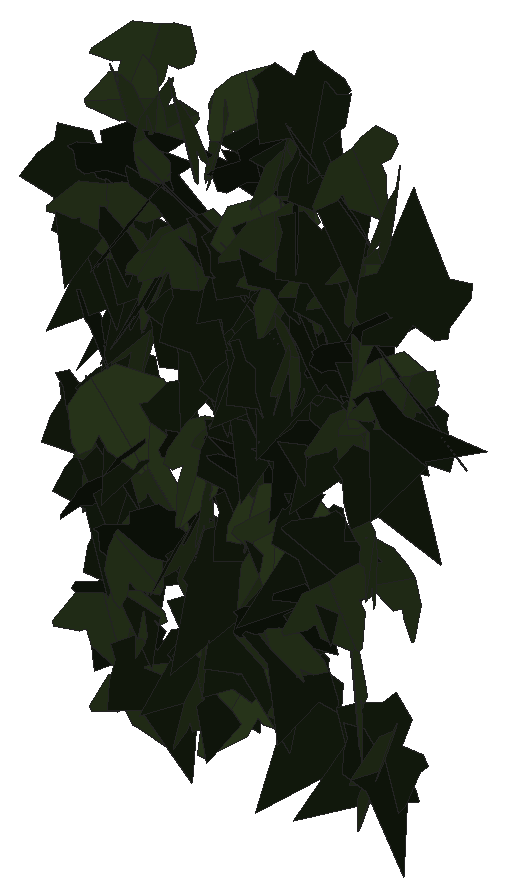
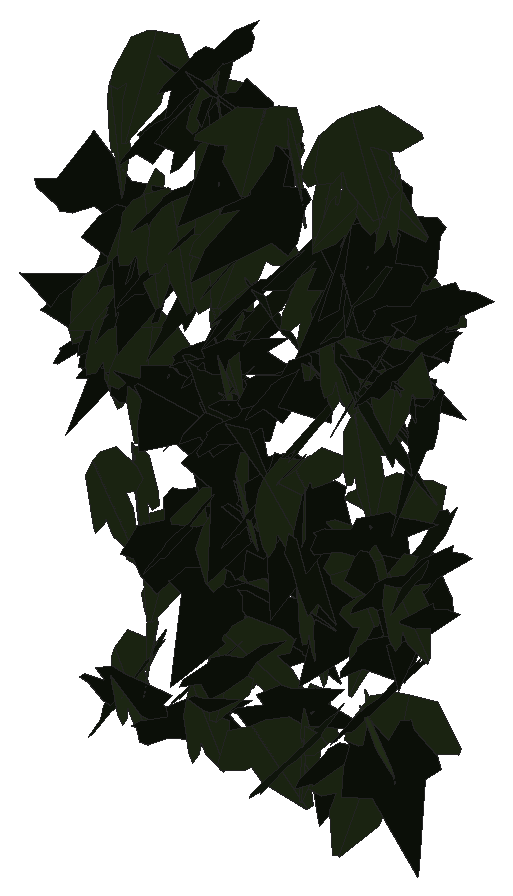
# SketchUp Ruby script. Lengths in inches.
U = 1.inch
M = Sketchup.active_model
def pt(a) = Geom::Point3d.new(a.map { |v| v * U })
def face(e, loops, mat)
  f = e.add_face(loops[0].map { |a| pt(a) })
  loops[1..].each { |l| e.add_face(l.map { |a| pt(a) }).erase! }
  f.material = f.back_material = mat if mat
  f
end
# faces: each face lists its corners as indices into pts; further lists are holes
def faces(e, pts, list, mat = nil) = list.each { |f| face(e, (f[0].is_a?(Array) ? f : [f]).map { |l| l.map { |i| pts[i] } }, mat) }
# xy, xz, yz: faces in a plane at the given z, y or x. An outline is a flat list of corners, or four numbers for a rectangle; further outlines are holes
def ring(l) = l.size == 4 ? [[l[0], l[1]], [l[2], l[1]], [l[2], l[3]], [l[0], l[3]]] : l.each_slice(2).to_a
def flat(e, list, mat, &to3) = list.each { |f| face(e, (f[0].is_a?(Array) ? f : [f]).map { |l| ring(l).map { |u, v| to3.(u, v) } }, mat) }
def xy(e, z, list, mat = nil) = flat(e, list, mat) { |x, y| [x, y, z] }
def xz(e, y, list, mat = nil) = flat(e, list, mat) { |x, z| [x, y, z] }
def yz(e, x, list, mat = nil) = flat(e, list, mat) { |y, z| [x, y, z] }
def lines(e, pts, list) = list.each { |a, b| e.add_line(pt(pts[a]), pt(pts[b])) }
# prism: a flat outline (further loops are holes) pulled along v
def prism(e, loops, v, mat = nil)
  f = face(e, loops, mat); d = Geom::Vector3d.new(v.map { |x| x * U })
  f.pushpull(f.normal.samedirection?(d) ? d.length : -d.length)
end
def box(e, o, s, mat = nil) = prism(e, [[o, [o[0] + s[0], o[1], o[2]], [o[0] + s[0], o[1] + s[1], o[2]], [o[0], o[1] + s[1], o[2]]]], [0, 0, s[2]], mat)
def at(x, y, z, deg = 0) = Geom::Transformation.translation(pt([x, y, z])) * Geom::Transformation.rotation(ORIGIN, Z_AXIS, deg.degrees)
def axes(o, x, y, z) = Geom::Transformation.new([*x, 0, *y, 0, *z, 0, *pt(o).to_a, 1])
def part(name) = M.definitions.add(name)
# library, detail: a bought-in or finely detailed component or shape, given as its bounding box
def library(name, o, s) = part(name).tap { |d| box(d.entities, o, s) }
def detail(e, o, s) = box(e.add_group.entities, o, s)
def put(e, d, t, mat = nil) = e.add_instance(d, t).tap { |i| i.material = mat if mat }
def group(e, t, mat = nil) = e.add_group.tap { |g| g.transformation = t; g.material = mat if mat }.entities
root = M.entities
M.materials.add("efeu1").color = [18, 25, 13]
M.materials.add("efeu2").color = [43, 57, 29]
c1 = part("ivyleaf_9")
p = [[1.54,2.16,1.25],[1.36,2.04,1.19],[-0.21,0.99,0.68],[-0.71,1.11,0.82],[-0.85,0.86,0.67],[-0.8,0.17,0.21],
  [-0.9,-0.01,0.1],[-0.67,-0.16,-0.02],[-0.08,-0.08,-0.05],[-0.03,-0.6,-0.4],[0.65,-0.88,-0.66],[0.83,-0.6,-0.49],
  [1.29,-0.42,-0.43],[1.8125,-0.07,-0.26],[1.21,0.44,0.15]]
faces(c1.entities,p,[[0,1,2,3,4,5,6,7,8,9,10,11,12,13,14]],"efeu1")
c2 = part("ivyleaf_10")
p = [[0,0.5,-0.03],[-0.0625,2.02,-0.43],[-0.19,2.01,-0.46],[-0.54,1.05,-0.29],[-0.52,0.625,-0.18],[-0.83,0.76,-0.28],
  [-1.16,0.64,-0.33],[-1.15,0.33,-0.24],[-0.77,-0.39,0.02],[-0.3,-0.51,0.16],[0.04,-0.48,0.23],[-0.02,2.01,-0.4375],
  [-0.06,2.01,-0.43],[0.04,-0.49,0.23],[0.67,-0.49,0.14],[1.38,0.36,-0.2],[1.375,0.51,-0.24],[0.81,0.65,-0.19],
  [0.62,0.59,-0.15],[0.6,1.09,-0.28],[0.5,1.23,-0.31]]
faces(c2.entities,p,[[0,1,2,3,4,5,6,7,8,9,10],[11,12,0,13,14,15,16,17,18,19,20]],"efeu2")
put(root,c1,axes([37.34,222.2,235.97],[0.37722,0.32248,0.06095],[0.04735,0.03841,-0.49627],[-0.32475,0.38018,-0.00156]))
put(root,c1,axes([39.04,222.6,238.55],[0.0869,-0.47634,-0.12469],[-0.01541,0.12393,-0.48415],[0.49215,0.08798,0.00686]))
put(root,c1,axes([37.5,222.54,239.24],[-0.33451,0.31048,-0.20422],[0.14578,-0.14311,-0.45636],[-0.34183,-0.36486,0.00522]))
put(root,c2,axes([38.09,222.62,237.15],[0.16547,0.41655,-0.22161],[-0.1056,-0.19618,-0.44762],[-0.45986,0.19494,0.02305]))
put(root,c1,axes([40.66,222.42,237.91],[0.16946,-0.36104,-0.30155],[-0.07838,0.29437,-0.39649],[0.46383,0.18165,0.04317]))
put(root,c2,axes([36.74,222.5,239.85],[-0.40261,-0.29647,0.00392],[0.00117,-0.00821,-0.49993],[0.29649,-0.40254,0.0073]))
put(root,c2,axes([37.23,222.22,235.65],[0.0086,0.38667,0.31687],[-0.10478,0.31128,-0.377],[-0.48882,-0.05992,0.08639]))
put(root,c2,axes([38.37,222.45,241.35],[0.27133,-0.37668,-0.18572],[-0.08916,0.16441,-0.4637],[0.4104,0.28475,0.02204]))
put(root,c1,axes([39.61,222.43,239.17],[0.39505,-0.24872,-0.17908],[-0.14662,0.10318,-0.46675],[0.26914,0.4213,0.00859]))
put(root,c2,axes([38.125,222.35,234.13],[0.10874,-0.40377,-0.27412],[-0.01169,0.27861,-0.41502],[0.48789,0.09667,0.05115]))
put(root,c2,axes([39.12,222.49,240.34],[-0.17321,-0.46244,-0.07843],[0.02367,0.07488,-0.49379],[0.46844,-0.17477,-0.00405]))
put(root,c2,axes([40.37,222.42,241.65],[-0.11075,-0.44868,-0.19083],[0.11484,0.16618,-0.45738],[0.47386,-0.14514,0.06625]))
put(root,c1,axes([36.92,222.25,240.7],[0.40628,0.28308,0.06933],[0.06105,0.03364,-0.49512],[-0.28498,0.41077,-0.00723]))
put(root,c1,axes([40.61,222.52,238.19],[0.21266,-0.11743,0.43702],[0.41769,-0.13484,-0.23948],[0.1741,0.46693,0.04075]))
put(root,c1,axes([40.4,222.76,233.83],[0.17251,-0.45623,0.10999],[0.03576,-0.10406,-0.48774],[0.46793,0.17614,-0.00327]))
put(root,c2,axes([39.03,222.8,236.26],[-0.06988,-0.40134,0.2899],[-0.00607,-0.29206,-0.40579],[0.49506,-0.06024,0.03594]))
put(root,c2,axes([39.41,222.4,241.38],[-0.05681,-0.43369,-0.24225],[0.04947,0.23768,-0.43711],[0.49429,-0.07364,0.01591]))
put(root,c1,axes([39.68,222.67,240.32],[0.09954,-0.48159,-0.09034],[0.01844,0.0958,-0.49039],[0.48964,0.09429,0.03683]))
put(root,c2,axes([36.76,222.375,237.33],[0.19447,0.40463,0.22012],[0.09816,0.19705,-0.44893],[-0.45005,0.21782,-0.0028]))
put(root,c2,axes([39.13,222.71,238.49],[0.25242,-0.4008,0.16013],[0.12288,-0.11109,-0.47176],[0.41374,0.27752,0.04242]))
put(root,c1,axes([37.42,222.52,240.34],[0.44373,-0.21345,0.08684],[0.08977,-0.01342,-0.49169],[0.21223,0.45195,0.02641]))
put(root,c1,axes([39.57,222.27,240.125],[-0.01123,-0.01698,0.49959],[-0.07321,0.49438,0.01516],[-0.49448,-0.07281,-0.01359]))
put(root,c1,axes([39.71,222.56,241.59],[-0.37062,0.22781,0.24646],[-0.25989,0.03753,-0.4255],[-0.21237,-0.4435,0.09059]))
put(root,c2,axes([40.32,222.65,239.87],[-0.04463,0.45966,-0.19163],[-0.02071,-0.19394,-0.46039],[-0.49757,-0.03315,0.03635]))
put(root,c2,axes([36.74,222.52,234.58],[-0.42381,-0.25499,-0.07323],[0.06664,0.03128,-0.49455],[0.25679,-0.42895,0.00748]))
put(root,c2,axes([39.26,222.58,241.52],[0.26271,-0.42076,-0.06279],[0.01411,0.08237,-0.49297],[0.42519,0.25725,0.05515]))
put(root,c1,axes([36.35,222.82,240.03],[-0.23638,-0.43841,-0.04384],[0.014,0.04225,-0.49801],[0.44037,-0.23667,-0.0077]))
put(root,c2,axes([36.92,222.56,241.24],[-0.39883,0.284,-0.10138],[0.06589,-0.08197,-0.48881],[-0.29427,-0.40326,0.02796]))
put(root,c2,axes([40.5,222.72,233.99],[0.14722,-0.46537,0.10846],[0.0319,-0.10366,-0.48809],[0.47677,0.15063,-0.00083]))
put(root,c1,axes([40.36,222.29,239.36],[0.19902,0.45709,0.03817],[0.01874,0.03347,-0.49853],[-0.4583,0.19987,-0.00381]))
put(root,c1,axes([39.84,222.77,241.19],[0.06856,-0.49467,-0.02444],[0.00004,0.02468,-0.49939],[0.49528,0.06848,0.00342]))
put(root,c1,axes([39.68,222.62,237.79],[0.00583,0.37533,-0.33029],[-0.00855,-0.33019,-0.37537],[-0.49989,0.01002,0.00257]))
put(root,c1,axes([38.86,222.67,239.91],[0.27997,-0.41382,-0.01935],[0.01716,0.03492,-0.49848],[0.41391,0.27846,0.03376]))
put(root,c2,axes([37.23,222.58,241.27],[-0.17263,0.06898,0.46415],[-0.46741,-0.06901,-0.16359],[0.04149,-0.49039,0.08831]))
put(root,c1,axes([36.84,222.33,236.4],[0.01588,0.49702,0.05215],[-0.00153,0.05222,-0.49726],[-0.49975,0.01564,0.00318]))
put(root,c1,axes([39.17,222.91,238.66],[-0.15747,-0.46524,0.09355],[-0.04715,-0.08274,-0.49085],[0.47221,-0.16341,-0.01782]))
put(root,c1,axes([37.14,222.47,239.75],[-0.20778,0.45365,-0.03204],[0.01801,-0.02699,-0.49895],[-0.45443,-0.2085,-0.00512]))
put(root,c2,axes([36.72,222.88,234.21],[0.01631,-0.17919,-0.4665],[0.284,-0.38073,0.15617],[-0.41119,-0.27007,0.08936]))
put(root,c1,axes([36.43,222.42,238.5625],[0.32565,-0.07045,-0.37281],[-0.35015,0.13338,-0.33106],[0.1461,0.4767,0.03753]))
put(root,c2,axes([38.16,222.48,236.71],[0.22087,-0.36723,-0.25761],[-0.03463,0.27232,-0.4179],[0.44723,0.20244,0.09486]))
put(root,c1,axes([40.73,222.97,238.28],[-0.1525,-0.45172,0.15065],[0.00501,-0.1597,-0.47378],[0.47615,-0.143,0.05323]))
put(root,c1,axes([39.36,222.73,241.42],[0.34639,-0.33329,0.13761],[0.09668,-0.09799,-0.48068],[0.34738,0.35961,-0.00344]))
put(root,c1,axes([38.32,222.82,235.5625],[-0.46652,-0.14953,-0.1],[0.09817,0.02129,-0.48981],[0.15074,-0.47664,0.00949]))
put(root,c2,axes([39.13,222.79,239.7],[-0.06086,-0.4689,0.16257],[-0.00375,-0.16335,-0.47255],[0.49627,-0.05874,0.01637]))
put(root,c2,axes([37.21,222.55,233.75],[-0.39639,-0.27136,-0.1387],[0.11431,0.07857,-0.48038],[0.2825,-0.41254,-0.00025]))
put(root,c1,axes([37.3,222.7,234.07],[0.04308,-0.45676,-0.19879],[-0.01847,0.19793,-0.45878],[0.4978,0.04687,0.00018]))
put(root,c2,axes([37.05,222.76,236.54],[-0.28719,0.06409,-0.40424],[0.34629,-0.2252,-0.28173],[-0.21818,-0.44179,0.08496]))
put(root,c2,axes([37.8,222.62,239.65],[-0.14338,-0.46754,-0.10414],[0.08401,0.08248,-0.48594],[0.47158,-0.15685,0.0549]))
put(root,c1,axes([37.97,222.74,236.4],[-0.3429,0.27146,-0.24234],[0.19342,-0.14609,-0.43732],[-0.30824,-0.39366,-0.00482]))
put(root,c1,axes([39.69,222.96,236.21],[-0.00788,0.02031,-0.49953],[0.00404,-0.49957,-0.02038],[-0.49992,-0.00436,0.0077]))
put(root,c2,axes([40.79,222.76,238.66],[-0.11898,-0.47885,0.08091],[0.0088,-0.08541,-0.49257],[0.48556,-0.11579,0.02875]))
put(root,c1,axes([36.93,222.91,239.15],[-0.43631,-0.21896,0.1081],[-0.10169,-0.03833,-0.48805],[0.22202,-0.44787,-0.01109]))
put(root,c1,axes([39.3,222.67,242.16],[0.1389,-0.42537,-0.22309],[-0.04129,0.22079,-0.44671],[0.47854,0.14251,0.02621]))
put(root,c1,axes([39.21,222.375,235.5],[0.32847,0.37544,0.03396],[0.0226,0.02535,-0.49884],[-0.37629,0.32925,-0.00032]))
put(root,c2,axes([39.02,222.67,236.61],[0.32281,0.38025,-0.03462],[-0.02507,-0.02413,-0.49879],[-0.381,0.32377,0.00349]))
put(root,c1,axes([37.29,222.79,239.13],[-0.37893,0.21297,-0.24709],[0.20005,-0.14743,-0.43387],[-0.25766,-0.42768,0.02652]))
put(root,c2,axes([39.9,222.58,235.84],[-0.22047,-0.4142,-0.17271],[0.09238,0.14641,-0.46907],[0.43915,-0.23875,0.01197]))
put(root,c1,axes([38.66,222.98,237.92],[-0.10477,-0.48173,0.08345],[-0.00717,-0.08382,-0.49287],[0.48885,-0.10447,0.01066]))
put(root,c1,axes([39.0625,223.04,234.59],[-0.05635,-0.42548,0.2565],[0.06493,-0.26224,-0.42073],[0.49255,-0.0141,0.08481]))
put(root,c1,axes([38.84,222.32,241.14],[0.29844,0.35343,0.18978],[0.10819,0.15687,-0.46226],[-0.3863,0.31698,0.01716]))
put(root,c2,axes([37.17,222.79,241.9],[-0.27441,-0.40092,0.11814],[-0.02693,-0.12408,-0.48361],[0.4171,-0.27178,0.0465]))
put(root,c2,axes([38.99,222.64,234.85],[-0.49242,-0.06286,-0.05974],[0.06029,-0.00057,-0.49635],[0.06233,-0.49603,0.00814]))
put(root,c2,axes([37.74,222.57,241.27],[-0.40403,0.27802,0.09728],[-0.08332,0.05051,-0.49042],[-0.28252,-0.4125,0.00551]))
put(root,c2,axes([37.28,222.9,239.21],[0.03757,-0.45391,0.20629],[0.08617,-0.19785,-0.45103],[0.49108,0.06944,0.06336]))
put(root,c2,axes([38.67,222.88,236.9375],[0.26323,-0.38075,0.18904],[0.11695,-0.1489,-0.46276],[0.40869,0.28785,0.01067]))
put(root,c1,axes([37.9375,222.89,238.68],[0.04543,-0.49611,-0.04258],[-0.0018,0.0426,-0.49818],[0.49793,0.04541,0.00209]))
put(root,c1,axes([38.33,222.92,236.99],[0.11122,-0.4865,0.03074],[-0.00033,-0.03161,-0.499],[0.48747,0.11098,-0.00735]))
put(root,c1,axes([38.9,222.66,238.18],[0.30711,-0.35585,-0.17044],[-0.02768,0.19603,-0.45914],[0.39359,0.29145,0.10071]))
put(root,c1,axes([39.03,223.07,238.57],[-0.35774,-0.31034,0.16036],[-0.06524,-0.16614,-0.46706],[0.34317,-0.35509,0.07838]))
put(root,c2,axes([38.78,222.74,234.84],[0.28578,-0.03867,-0.40846],[-0.40443,0.05722,-0.28838],[0.06905,0.49521,0.00143]))
put(root,c2,axes([40,222.89,234.71],[-0.24239,0.31226,-0.30617],[0.1188,-0.28987,-0.38969],[-0.42087,-0.26166,0.06633]))
put(root,c1,axes([36.15,222.84,236.96],[0.30388,-0.3962,0.02621],[0.01686,-0.0201,-0.49931],[0.3967,0.30434,0.00115]))
put(root,c2,axes([39.31,222.52,238.7],[0.2008,-0.11641,-0.44287],[-0.27872,0.35261,-0.21905],[0.36332,0.33484,0.07672]))
put(root,c1,axes([38.71,222.51,237.125],[0.38675,0.3094,-0.06852],[-0.05032,-0.04678,-0.49526],[-0.31288,0.38998,-0.00505]))
put(root,c1,axes([38.02,223.01,238.67],[-0.25676,-0.42903,0.00187],[-0.00086,-0.00166,-0.5],[0.42904,-0.25676,0.00011]))
put(root,c2,axes([40.61,222.74,241.0625],[0.18642,-0.45388,-0.09614],[0.00079,0.10392,-0.48908],[0.46395,0.1822,0.03946]))
put(root,c1,axes([38.1875,223.08,234.48],[-0.39891,-0.25095,0.16702],[-0.10574,-0.14294,-0.46732],[0.2823,-0.40816,0.06097]))
put(root,c2,axes([37.81,222.78,235.86],[0.1179,-0.48334,-0.04977],[-0.00998,0.04879,-0.49751],[0.4858,0.11831,0.00186]))
put(root,c1,axes([37.88,223.12,233.86],[-0.03575,-0.41634,0.27456],[0.08878,-0.27618,-0.40724],[0.49075,0.01963,0.09367]))
put(root,c1,axes([37.22,222.97,239.04],[-0.4626,-0.16189,-0.09894],[0.10337,0.00358,-0.48918],[0.1591,-0.47305,0.03016]))
put(root,c2,axes([39.68,222.82,239.91],[-0.07293,-0.49448,0.01309],[0.00134,-0.01343,-0.49982],[0.49465,-0.07287,0.00329]))
put(root,c1,axes([39.73,222.99,239.54],[0.07112,-0.49399,0.03025],[0.00284,-0.03016,-0.49908],[0.49491,0.07116,-0.00149]))
put(root,c1,axes([37.99,222.6,237.01],[0.41672,0.20409,-0.18626],[-0.16096,-0.09465,-0.46383],[-0.22459,0.44653,-0.01319]))
put(root,c1,axes([37.49,222.83,238.38],[0.27273,-0.41435,-0.06275],[-0.00762,0.06995,-0.49502],[0.419,0.27097,0.03184]))
put(root,c1,axes([38.63,222.86,236.38],[-0.20635,-0.18601,-0.41572],[0.37015,0.19741,-0.27206],[0.26534,-0.42004,0.05623]))
put(root,c1,axes([40.5,222.97,233.89],[-0.49075,-0.04414,0.08493],[-0.08226,-0.03237,-0.49212],[0.04895,-0.49699,0.02451]))
put(root,c1,axes([37.07,223,239.9],[0.18277,-0.4055,0.2284],[0.19397,-0.15668,-0.43339],[0.42305,0.24703,0.10004]))
put(root,c2,axes([37.41,222.41,240.87],[0.00029,0.0621,0.49613],[-0.16369,0.4688,-0.05858],[-0.47245,-0.16239,0.0206]))
put(root,c1,axes([38.08,222.87,239.66],[0.2849,-0.41075,-0.01071],[0.03693,0.03858,-0.49714],[0.40923,0.28248,0.05232]))
put(root,c2,axes([40.31,222.7,236.55],[0.35716,-0.29326,-0.19088],[-0.06017,0.21723,-0.44631],[0.3447,0.34178,0.11988]))
put(root,c1,axes([36.33,223.01,239.42],[0.0275,-0.49921,-0.00537],[0.01281,0.00609,-0.4998],[0.49908,0.02735,0.01312]))
put(root,c2,axes([40.12,222.74,238.13],[-0.17779,-0.45108,-0.12215],[0.04456,0.11373,-0.48485],[0.46519,-0.18329,-0.00024]))
put(root,c1,axes([38.48,222.8125,239.39],[-0.43538,0.2451,0.01917],[-0.01777,0.00752,-0.49963],[-0.2452,-0.43574,0.00216]))
put(root,c1,axes([38.65,222.94,236.29],[-0.02593,-0.0301,0.49842],[0.3458,-0.36112,-0.00382],[0.36021,0.34451,0.03954]))
put(root,c2,axes([40.48,222.74,238.6875],[0.13757,0.48038,0.01769],[-0.02874,0.02659,-0.49846],[-0.47984,0.13613,0.03493]))
put(root,c2,axes([40.46,222.88,238.4],[-0.08223,-0.49244,0.0272],[0.09157,-0.04234,-0.48972],[0.48462,-0.07556,0.09715]))
put(root,c1,axes([40.95,222.6875,239.69],[-0.44958,-0.10113,0.19403],[0.1897,0.0408,0.46081],[-0.10903,0.48796,0.00168]))
put(root,c1,axes([36.3,223.01,236.74],[-0.04469,-0.49375,-0.0649],[0.03703,0.06169,-0.4948],[0.49662,-0.04903,0.03105]))
put(root,c1,axes([40.52,222.93,238.77],[0.34847,-0.3079,0.18376],[0.13204,-0.12805,-0.46494],[0.33337,0.37256,-0.00793]))
put(root,c1,axes([39.5,223.15,233.89],[-0.345,-0.34069,0.1221],[-0.05334,-0.11898,-0.4827],[0.35795,-0.34609,0.04575]))
put(root,c2,axes([38.7,222.82,240.16],[-0.3176,-0.36,-0.13975],[0.20218,-0.00085,-0.4573],[0.32902,-0.34699,0.14611]))
put(root,c1,axes([38.65,222.96,234.84],[-0.0652,-0.46504,-0.17173],[0.09295,0.15867,-0.46496],[0.48694,-0.09255,0.06576]))
put(root,c1,axes([39.33,223.05,236.36],[0.09072,-0.48906,0.0509],[0.00495,-0.05085,-0.49738],[0.49168,0.09075,-0.00438]))
put(root,c1,axes([36.72,222.64,239.61],[0.33654,-0.18224,-0.32176],[-0.23461,0.23106,-0.37625],[0.28583,0.40423,0.07001]))
put(root,c2,axes([36.375,223.02,236.53],[0.10036,-0.46251,0.16129],[0.04097,-0.15614,-0.47323],[0.48811,0.1082,0.00655]))
put(root,c2,axes([37.28,222.94,239.32],[0.03578,-0.49509,0.06002],[0.01507,-0.05908,-0.49627],[0.49849,0.03733,0.0107]))
put(root,c2,axes([38.1,223.06,237.15],[0.05108,-0.44598,0.22021],[0.05239,-0.21531,-0.44821],[0.49462,0.06887,0.02473]))
put(root,c2,axes([39.17,223.03,234.15],[0.07524,-0.46023,0.18036],[0.08502,-0.16767,-0.46331],[0.48694,0.10039,0.05302]))
put(root,c2,axes([40.04,222.875,239.89],[-0.08219,-0.49286,-0.01835],[-0.00933,0.02015,-0.49951],[0.49311,-0.08177,-0.01251]))
put(root,c1,axes([38.71,222.99,238.08],[-0.01105,-0.48354,-0.12674],[-0.00078,0.12679,-0.48366],[0.49988,-0.01049,-0.00356]))
put(root,c1,axes([36.63,223.0625,235.11],[0.09096,-0.4912,0.02126],[0.03043,-0.01596,-0.49882],[0.49071,0.09204,0.02699]))
put(root,c1,axes([36.84,222.62,240.31],[0.45356,0.19919,0.06786],[0.06361,0.0239,-0.49536],[-0.20059,0.45799,-0.00366]))
put(root,c1,axes([36.91,223.16,237.17],[-0.31784,-0.38588,0.00857],[0.03177,-0.03721,-0.4976],[0.38467,-0.31577,0.04817]))
put(root,c1,axes([38.37,222.68,240.77],[0.49454,0.07208,-0.01535],[-0.01739,0.01295,-0.49953],[-0.07161,0.49461,0.01531]))
put(root,c2,axes([36.64,222.79,239.27],[-0.49133,0.06154,0.06931],[-0.06742,0.01924,-0.49506],[-0.0636,-0.49583,-0.0106]))
put(root,c1,axes([36.4375,223.12,235.97],[-0.09208,-0.49126,-0.01364],[-0.00275,0.01439,-0.49979],[0.49144,-0.09196,-0.00535]))
put(root,c2,axes([40.78,222.71,236.26],[0.27426,-0.05192,-0.41483],[-0.31816,0.29593,-0.24739],[0.27121,0.39966,0.12929]))
put(root,c1,axes([39.22,222.83,238.18],[-0.3514,0.35567,0.00365],[-0.00295,0.00222,-0.49999],[-0.35568,-0.35141,0.00054]))
put(root,c1,axes([39.9,223.125,238],[-0.44402,-0.2287,-0.02339],[0.02221,0.00796,-0.49944],[0.22881,-0.44456,0.00309]))
put(root,c1,axes([36.84,223.01,238.71],[-0.42338,0.19251,-0.18355],[0.1568,-0.09809,-0.46454],[-0.21487,-0.45091,0.02269]))
put(root,c1,axes([38.38,222.91,239.69],[0.20493,-0.42096,-0.17549],[0.00006,0.19241,-0.46149],[0.45608,0.18912,0.07891]))
put(root,c2,axes([38.3125,222.99,233.96],[0.41583,0.19081,-0.20168],[-0.18846,-0.07273,-0.45738],[-0.20388,0.4564,0.01143]))
put(root,c2,axes([36.99,222.94,238.22],[0.07284,-0.49137,-0.05701],[-0.01476,0.05544,-0.4967],[0.49445,0.07404,-0.00643]))
put(root,c1,axes([36.68,222.84,234.38],[0.23915,0.15964,-0.40905],[-0.36819,-0.1809,-0.28586],[-0.23926,0.43794,0.03104]))
put(root,c2,axes([38.49,222.85,241.63],[0.26628,0.41441,0.08577],[0.03948,0.07657,-0.49252],[-0.42135,0.26907,0.00805]))
